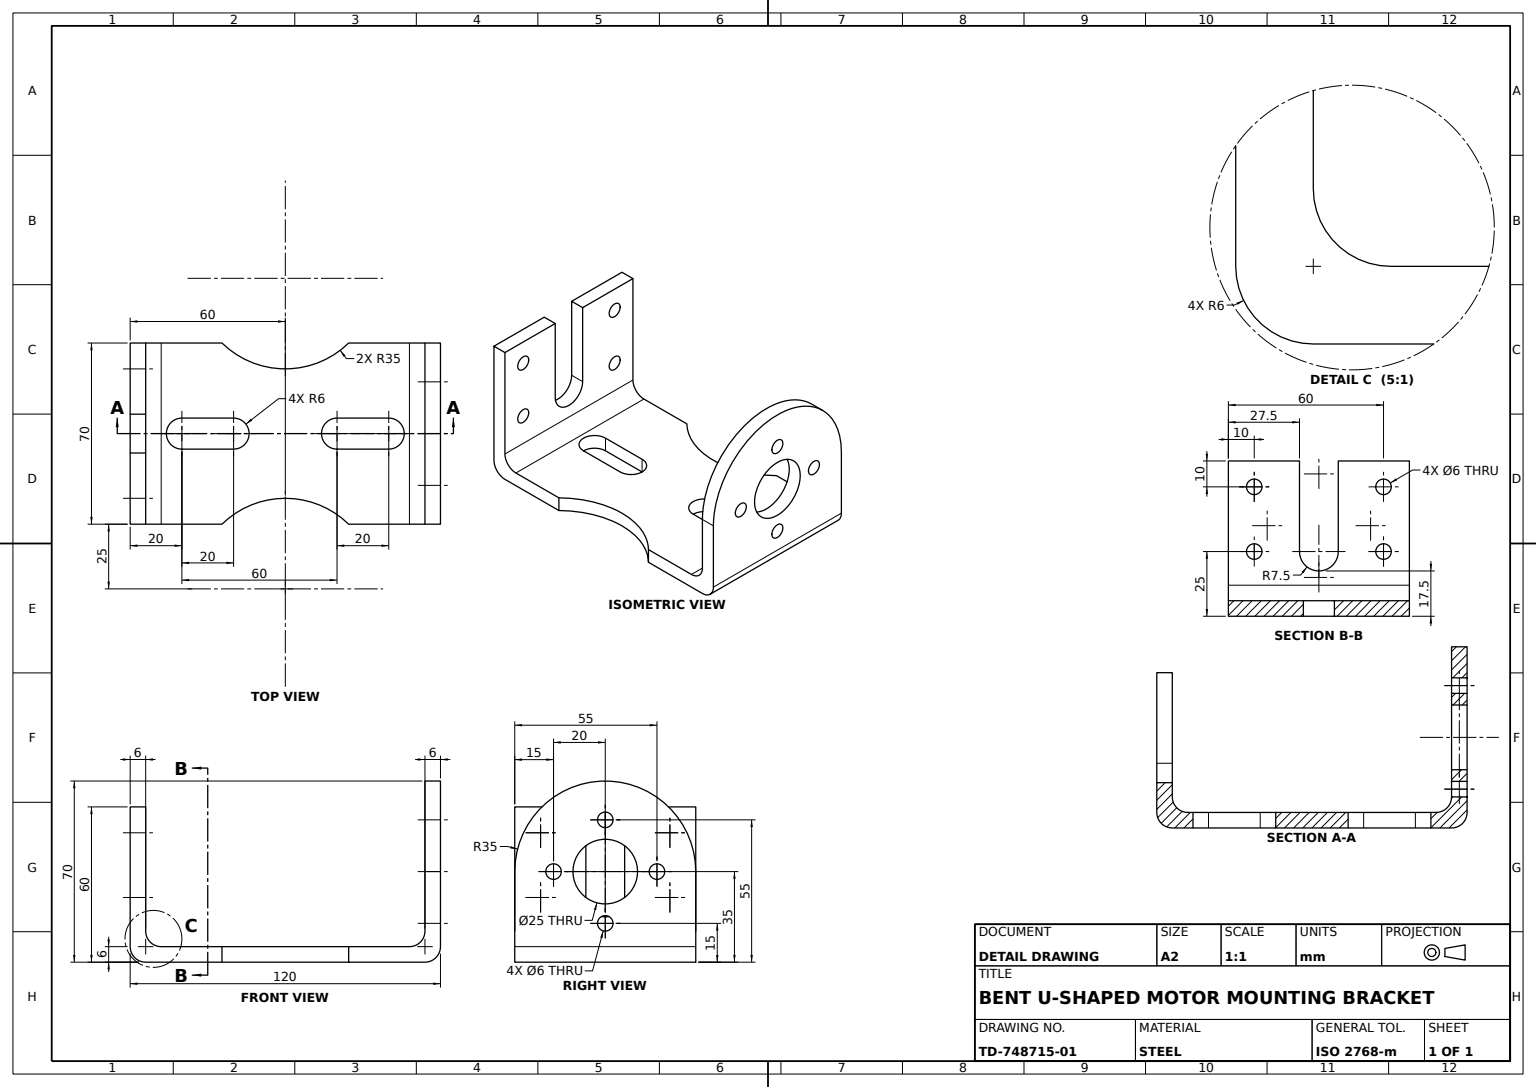
ISO-10303-21;
HEADER;
FILE_DESCRIPTION((''),'2;1');
FILE_NAME('','',(''),(''),'','','');
FILE_SCHEMA(('AUTOMOTIVE_DESIGN'));
ENDSEC;
DATA;
#1=APPLICATION_CONTEXT('');
#2=PRODUCT_CONTEXT('',#1,'mechanical');
#3=PRODUCT('','','',(#2));
#4=PRODUCT_DEFINITION_FORMATION('','',#3);
#5=PRODUCT_DEFINITION_CONTEXT('',#1,'design');
#6=PRODUCT_DEFINITION('','',#4,#5);
#7=PRODUCT_DEFINITION_SHAPE('','',#6);
#8=(LENGTH_UNIT()NAMED_UNIT(*)SI_UNIT(.MILLI.,.METRE.));
#9=(NAMED_UNIT(*)PLANE_ANGLE_UNIT()SI_UNIT($,.RADIAN.));
#10=(NAMED_UNIT(*)SI_UNIT($,.STERADIAN.)SOLID_ANGLE_UNIT());
#11=UNCERTAINTY_MEASURE_WITH_UNIT(LENGTH_MEASURE(1.E-05),#8,'distance_accuracy_value','');
#12=(GEOMETRIC_REPRESENTATION_CONTEXT(3)GLOBAL_UNCERTAINTY_ASSIGNED_CONTEXT((#11))GLOBAL_UNIT_ASSIGNED_CONTEXT((#8,#9,#10))REPRESENTATION_CONTEXT('',''));
#13=CARTESIAN_POINT('',(-20.,0.,6.));
#14=VERTEX_POINT('',#13);
#15=CARTESIAN_POINT('',(-20.,0.,-6.));
#16=VERTEX_POINT('',#15);
#17=CARTESIAN_POINT('',(-20.,0.,0.));
#18=DIRECTION('',(0.,1.,0.));
#19=DIRECTION('',(0.,0.,1.));
#20=AXIS2_PLACEMENT_3D('',#17,#18,#19);
#21=CIRCLE('',#20,6.);
#22=EDGE_CURVE('',#14,#16,#21,.T.);
#23=ORIENTED_EDGE('',*,*,#22,.T.);
#24=CARTESIAN_POINT('',(-40.,0.,-6.));
#25=VERTEX_POINT('',#24);
#26=DIRECTION('',(-1.,0.,0.));
#27=VECTOR('',#26,1000.);
#28=LINE('',#24,#27);
#29=EDGE_CURVE('',#16,#25,#28,.T.);
#30=ORIENTED_EDGE('',*,*,#29,.T.);
#31=CARTESIAN_POINT('',(-40.,0.,6.));
#32=VERTEX_POINT('',#31);
#33=CARTESIAN_POINT('',(-40.,0.,0.));
#34=AXIS2_PLACEMENT_3D('',#33,#18,#19);
#35=CIRCLE('',#34,6.);
#36=EDGE_CURVE('',#25,#32,#35,.T.);
#37=ORIENTED_EDGE('',*,*,#36,.T.);
#38=DIRECTION('',(1.,0.,0.));
#39=VECTOR('',#38,1000.);
#40=LINE('',#31,#39);
#41=EDGE_CURVE('',#32,#14,#40,.T.);
#42=ORIENTED_EDGE('',*,*,#41,.T.);
#43=EDGE_LOOP('',(#23,#30,#37,#42));
#44=FACE_BOUND('',#43,.T.);
#45=CARTESIAN_POINT('',(-54.,0.,35.));
#46=VERTEX_POINT('',#45);
#47=CARTESIAN_POINT('',(-24.494897,0.,35.));
#48=VERTEX_POINT('',#47);
#49=CARTESIAN_POINT('',(-60.,0.,35.));
#50=LINE('',#49,#39);
#51=EDGE_CURVE('',#46,#48,#50,.T.);
#52=ORIENTED_EDGE('',*,*,#51,.F.);
#53=CARTESIAN_POINT('',(-54.,0.,-35.));
#54=VERTEX_POINT('',#53);
#55=CARTESIAN_POINT('',(-54.,0.,60.));
#56=DIRECTION('',(0.,0.,-1.));
#57=VECTOR('',#56,1000.);
#58=LINE('',#55,#57);
#59=EDGE_CURVE('',#46,#54,#58,.T.);
#60=ORIENTED_EDGE('',*,*,#59,.T.);
#61=CARTESIAN_POINT('',(-24.494897,0.,-35.));
#62=VERTEX_POINT('',#61);
#63=CARTESIAN_POINT('',(-60.,0.,-35.));
#64=LINE('',#63,#27);
#65=EDGE_CURVE('',#62,#54,#64,.T.);
#66=ORIENTED_EDGE('',*,*,#65,.F.);
#67=CARTESIAN_POINT('',(24.494897,0.,-35.));
#68=VERTEX_POINT('',#67);
#69=CARTESIAN_POINT('',(0.,0.,-60.));
#70=DIRECTION('',(0.,-1.,0.));
#71=AXIS2_PLACEMENT_3D('',#69,#70,#19);
#72=CIRCLE('',#71,35.);
#73=EDGE_CURVE('',#68,#62,#72,.T.);
#74=ORIENTED_EDGE('',*,*,#73,.F.);
#75=CARTESIAN_POINT('',(54.,0.,-35.));
#76=VERTEX_POINT('',#75);
#77=LINE('',#67,#27);
#78=EDGE_CURVE('',#76,#68,#77,.T.);
#79=ORIENTED_EDGE('',*,*,#78,.F.);
#80=CARTESIAN_POINT('',(54.,0.,35.));
#81=VERTEX_POINT('',#80);
#82=CARTESIAN_POINT('',(54.,0.,60.));
#83=VECTOR('',#19,1000.);
#84=LINE('',#82,#83);
#85=EDGE_CURVE('',#76,#81,#84,.T.);
#86=ORIENTED_EDGE('',*,*,#85,.T.);
#87=CARTESIAN_POINT('',(24.494897,0.,35.));
#88=VERTEX_POINT('',#87);
#89=LINE('',#87,#39);
#90=EDGE_CURVE('',#88,#81,#89,.T.);
#91=ORIENTED_EDGE('',*,*,#90,.F.);
#92=CARTESIAN_POINT('',(0.,0.,25.));
#93=VERTEX_POINT('',#92);
#94=CARTESIAN_POINT('',(0.,0.,60.));
#95=AXIS2_PLACEMENT_3D('',#94,#70,#19);
#96=CIRCLE('',#95,35.);
#97=EDGE_CURVE('',#93,#88,#96,.T.);
#98=ORIENTED_EDGE('',*,*,#97,.F.);
#99=EDGE_CURVE('',#48,#93,#96,.T.);
#100=ORIENTED_EDGE('',*,*,#99,.F.);
#101=EDGE_LOOP('',(#52,#60,#66,#74,#79,#86,#91,#98,#100));
#102=FACE_OUTER_BOUND('',#101,.T.);
#103=CARTESIAN_POINT('',(20.,0.,6.));
#104=VERTEX_POINT('',#103);
#105=CARTESIAN_POINT('',(40.,0.,6.));
#106=VERTEX_POINT('',#105);
#107=LINE('',#103,#39);
#108=EDGE_CURVE('',#104,#106,#107,.T.);
#109=ORIENTED_EDGE('',*,*,#108,.T.);
#110=CARTESIAN_POINT('',(40.,0.,-6.));
#111=VERTEX_POINT('',#110);
#112=CARTESIAN_POINT('',(40.,0.,0.));
#113=AXIS2_PLACEMENT_3D('',#112,#18,#19);
#114=CIRCLE('',#113,6.);
#115=EDGE_CURVE('',#106,#111,#114,.T.);
#116=ORIENTED_EDGE('',*,*,#115,.T.);
#117=CARTESIAN_POINT('',(20.,0.,-6.));
#118=VERTEX_POINT('',#117);
#119=LINE('',#117,#27);
#120=EDGE_CURVE('',#111,#118,#119,.T.);
#121=ORIENTED_EDGE('',*,*,#120,.T.);
#122=CARTESIAN_POINT('',(20.,0.,0.));
#123=AXIS2_PLACEMENT_3D('',#122,#18,#19);
#124=CIRCLE('',#123,6.);
#125=EDGE_CURVE('',#118,#104,#124,.T.);
#126=ORIENTED_EDGE('',*,*,#125,.T.);
#127=EDGE_LOOP('',(#109,#116,#121,#126));
#128=FACE_BOUND('',#127,.T.);
#129=AXIS2_PLACEMENT_3D('',#94,#18,#19);
#130=PLANE('',#129);
#131=ADVANCED_FACE('',(#44,#102,#128),#130,.F.);
#132=CARTESIAN_POINT('',(60.,35.,-12.5));
#133=VERTEX_POINT('',#132);
#134=CARTESIAN_POINT('',(60.,35.,12.5));
#135=VERTEX_POINT('',#134);
#136=CARTESIAN_POINT('',(60.,35.,0.));
#137=AXIS2_PLACEMENT_3D('',#136,#38,#56);
#138=CIRCLE('',#137,12.5);
#139=EDGE_CURVE('',#133,#135,#138,.T.);
#140=ORIENTED_EDGE('',*,*,#139,.T.);
#141=CARTESIAN_POINT('',(54.,35.,12.5));
#142=VERTEX_POINT('',#141);
#143=LINE('',#141,#39);
#144=EDGE_CURVE('',#142,#135,#143,.T.);
#145=ORIENTED_EDGE('',*,*,#144,.F.);
#146=CARTESIAN_POINT('',(54.,35.,-12.5));
#147=VERTEX_POINT('',#146);
#148=CARTESIAN_POINT('',(54.,35.,0.));
#149=AXIS2_PLACEMENT_3D('',#148,#38,#56);
#150=CIRCLE('',#149,12.5);
#151=EDGE_CURVE('',#147,#142,#150,.T.);
#152=ORIENTED_EDGE('',*,*,#151,.F.);
#153=LINE('',#146,#39);
#154=EDGE_CURVE('',#147,#133,#153,.T.);
#155=ORIENTED_EDGE('',*,*,#154,.T.);
#156=EDGE_LOOP('',(#140,#145,#152,#155));
#157=FACE_OUTER_BOUND('',#156,.T.);
#158=CYLINDRICAL_SURFACE('',#149,12.5);
#159=ADVANCED_FACE('',(#157),#158,.F.);
#160=CARTESIAN_POINT('',(-40.,6.,-6.));
#161=VERTEX_POINT('',#160);
#162=CARTESIAN_POINT('',(-40.,6.,6.));
#163=VERTEX_POINT('',#162);
#164=CARTESIAN_POINT('',(-40.,6.,0.));
#165=AXIS2_PLACEMENT_3D('',#164,#18,#19);
#166=CIRCLE('',#165,6.);
#167=EDGE_CURVE('',#161,#163,#166,.T.);
#168=ORIENTED_EDGE('',*,*,#167,.T.);
#169=VECTOR('',#70,1000.);
#170=LINE('',#162,#169);
#171=EDGE_CURVE('',#163,#32,#170,.T.);
#172=ORIENTED_EDGE('',*,*,#171,.T.);
#173=ORIENTED_EDGE('',*,*,#36,.F.);
#174=LINE('',#160,#169);
#175=EDGE_CURVE('',#161,#25,#174,.T.);
#176=ORIENTED_EDGE('',*,*,#175,.F.);
#177=EDGE_LOOP('',(#168,#172,#173,#176));
#178=FACE_OUTER_BOUND('',#177,.T.);
#179=AXIS2_PLACEMENT_3D('',#164,#70,#56);
#180=CYLINDRICAL_SURFACE('',#179,6.);
#181=ADVANCED_FACE('',(#178),#180,.F.);
#182=CARTESIAN_POINT('',(54.,35.,-23.));
#183=VERTEX_POINT('',#182);
#184=CARTESIAN_POINT('',(54.,35.,-17.));
#185=VERTEX_POINT('',#184);
#186=CARTESIAN_POINT('',(54.,35.,-20.));
#187=AXIS2_PLACEMENT_3D('',#186,#38,#56);
#188=CIRCLE('',#187,3.);
#189=EDGE_CURVE('',#183,#185,#188,.T.);
#190=ORIENTED_EDGE('',*,*,#189,.F.);
#191=CARTESIAN_POINT('',(60.,35.,-23.));
#192=VERTEX_POINT('',#191);
#193=LINE('',#182,#39);
#194=EDGE_CURVE('',#183,#192,#193,.T.);
#195=ORIENTED_EDGE('',*,*,#194,.T.);
#196=CARTESIAN_POINT('',(60.,35.,-17.));
#197=VERTEX_POINT('',#196);
#198=CARTESIAN_POINT('',(60.,35.,-20.));
#199=AXIS2_PLACEMENT_3D('',#198,#38,#56);
#200=CIRCLE('',#199,3.);
#201=EDGE_CURVE('',#192,#197,#200,.T.);
#202=ORIENTED_EDGE('',*,*,#201,.T.);
#203=LINE('',#184,#39);
#204=EDGE_CURVE('',#185,#197,#203,.T.);
#205=ORIENTED_EDGE('',*,*,#204,.F.);
#206=EDGE_LOOP('',(#190,#195,#202,#205));
#207=FACE_OUTER_BOUND('',#206,.T.);
#208=CYLINDRICAL_SURFACE('',#187,3.);
#209=ADVANCED_FACE('',(#207),#208,.F.);
#210=CARTESIAN_POINT('',(-60.,50.,22.));
#211=VERTEX_POINT('',#210);
#212=CARTESIAN_POINT('',(-60.,50.,28.));
#213=VERTEX_POINT('',#212);
#214=CARTESIAN_POINT('',(-60.,50.,25.));
#215=AXIS2_PLACEMENT_3D('',#214,#26,#19);
#216=CIRCLE('',#215,3.);
#217=EDGE_CURVE('',#211,#213,#216,.T.);
#218=ORIENTED_EDGE('',*,*,#217,.T.);
#219=CARTESIAN_POINT('',(-54.,50.,28.));
#220=VERTEX_POINT('',#219);
#221=LINE('',#219,#27);
#222=EDGE_CURVE('',#220,#213,#221,.T.);
#223=ORIENTED_EDGE('',*,*,#222,.F.);
#224=CARTESIAN_POINT('',(-54.,50.,22.));
#225=VERTEX_POINT('',#224);
#226=CARTESIAN_POINT('',(-54.,50.,25.));
#227=AXIS2_PLACEMENT_3D('',#226,#26,#19);
#228=CIRCLE('',#227,3.);
#229=EDGE_CURVE('',#225,#220,#228,.T.);
#230=ORIENTED_EDGE('',*,*,#229,.F.);
#231=LINE('',#224,#27);
#232=EDGE_CURVE('',#225,#211,#231,.T.);
#233=ORIENTED_EDGE('',*,*,#232,.T.);
#234=EDGE_LOOP('',(#218,#223,#230,#233));
#235=FACE_OUTER_BOUND('',#234,.T.);
#236=CYLINDRICAL_SURFACE('',#227,3.);
#237=ADVANCED_FACE('',(#235),#236,.F.);
#238=CARTESIAN_POINT('',(20.,6.,6.));
#239=VERTEX_POINT('',#238);
#240=LINE('',#238,#169);
#241=EDGE_CURVE('',#239,#104,#240,.T.);
#242=ORIENTED_EDGE('',*,*,#241,.T.);
#243=ORIENTED_EDGE('',*,*,#125,.F.);
#244=CARTESIAN_POINT('',(20.,6.,-6.));
#245=VERTEX_POINT('',#244);
#246=LINE('',#244,#169);
#247=EDGE_CURVE('',#245,#118,#246,.T.);
#248=ORIENTED_EDGE('',*,*,#247,.F.);
#249=CARTESIAN_POINT('',(20.,6.,0.));
#250=AXIS2_PLACEMENT_3D('',#249,#18,#19);
#251=CIRCLE('',#250,6.);
#252=EDGE_CURVE('',#245,#239,#251,.T.);
#253=ORIENTED_EDGE('',*,*,#252,.T.);
#254=EDGE_LOOP('',(#242,#243,#248,#253));
#255=FACE_OUTER_BOUND('',#254,.T.);
#256=AXIS2_PLACEMENT_3D('',#249,#70,#56);
#257=CYLINDRICAL_SURFACE('',#256,6.);
#258=ADVANCED_FACE('',(#255),#257,.F.);
#259=CARTESIAN_POINT('',(60.,55.,3.));
#260=VERTEX_POINT('',#259);
#261=CARTESIAN_POINT('',(60.,55.,-3.));
#262=VERTEX_POINT('',#261);
#263=CARTESIAN_POINT('',(60.,55.,0.));
#264=AXIS2_PLACEMENT_3D('',#263,#38,#56);
#265=CIRCLE('',#264,3.);
#266=EDGE_CURVE('',#260,#262,#265,.T.);
#267=ORIENTED_EDGE('',*,*,#266,.T.);
#268=CARTESIAN_POINT('',(54.,55.,-3.));
#269=VERTEX_POINT('',#268);
#270=LINE('',#268,#39);
#271=EDGE_CURVE('',#269,#262,#270,.T.);
#272=ORIENTED_EDGE('',*,*,#271,.F.);
#273=CARTESIAN_POINT('',(54.,55.,3.));
#274=VERTEX_POINT('',#273);
#275=CARTESIAN_POINT('',(54.,55.,0.));
#276=AXIS2_PLACEMENT_3D('',#275,#38,#56);
#277=CIRCLE('',#276,3.);
#278=EDGE_CURVE('',#274,#269,#277,.T.);
#279=ORIENTED_EDGE('',*,*,#278,.F.);
#280=LINE('',#273,#39);
#281=EDGE_CURVE('',#274,#260,#280,.T.);
#282=ORIENTED_EDGE('',*,*,#281,.T.);
#283=EDGE_LOOP('',(#267,#272,#279,#282));
#284=FACE_OUTER_BOUND('',#283,.T.);
#285=CYLINDRICAL_SURFACE('',#276,3.);
#286=ADVANCED_FACE('',(#284),#285,.F.);
#287=CARTESIAN_POINT('',(-54.,25.,22.));
#288=VERTEX_POINT('',#287);
#289=CARTESIAN_POINT('',(-60.,25.,22.));
#290=VERTEX_POINT('',#289);
#291=LINE('',#287,#27);
#292=EDGE_CURVE('',#288,#290,#291,.T.);
#293=ORIENTED_EDGE('',*,*,#292,.T.);
#294=CARTESIAN_POINT('',(-60.,25.,28.));
#295=VERTEX_POINT('',#294);
#296=CARTESIAN_POINT('',(-60.,25.,25.));
#297=AXIS2_PLACEMENT_3D('',#296,#26,#19);
#298=CIRCLE('',#297,3.);
#299=EDGE_CURVE('',#290,#295,#298,.T.);
#300=ORIENTED_EDGE('',*,*,#299,.T.);
#301=CARTESIAN_POINT('',(-54.,25.,28.));
#302=VERTEX_POINT('',#301);
#303=LINE('',#301,#27);
#304=EDGE_CURVE('',#302,#295,#303,.T.);
#305=ORIENTED_EDGE('',*,*,#304,.F.);
#306=CARTESIAN_POINT('',(-54.,25.,25.));
#307=AXIS2_PLACEMENT_3D('',#306,#26,#19);
#308=CIRCLE('',#307,3.);
#309=EDGE_CURVE('',#288,#302,#308,.T.);
#310=ORIENTED_EDGE('',*,*,#309,.F.);
#311=EDGE_LOOP('',(#293,#300,#305,#310));
#312=FACE_OUTER_BOUND('',#311,.T.);
#313=CYLINDRICAL_SURFACE('',#307,3.);
#314=ADVANCED_FACE('',(#312),#313,.F.);
#315=EDGE_CURVE('',#220,#225,#228,.T.);
#316=ORIENTED_EDGE('',*,*,#315,.F.);
#317=ORIENTED_EDGE('',*,*,#222,.T.);
#318=EDGE_CURVE('',#213,#211,#216,.T.);
#319=ORIENTED_EDGE('',*,*,#318,.T.);
#320=ORIENTED_EDGE('',*,*,#232,.F.);
#321=EDGE_LOOP('',(#316,#317,#319,#320));
#322=FACE_OUTER_BOUND('',#321,.T.);
#323=ADVANCED_FACE('',(#322),#236,.F.);
#324=ORIENTED_EDGE('',*,*,#292,.F.);
#325=EDGE_CURVE('',#302,#288,#308,.T.);
#326=ORIENTED_EDGE('',*,*,#325,.F.);
#327=ORIENTED_EDGE('',*,*,#304,.T.);
#328=EDGE_CURVE('',#295,#290,#298,.T.);
#329=ORIENTED_EDGE('',*,*,#328,.T.);
#330=EDGE_LOOP('',(#324,#326,#327,#329));
#331=FACE_OUTER_BOUND('',#330,.T.);
#332=ADVANCED_FACE('',(#331),#313,.F.);
#333=CARTESIAN_POINT('',(-60.,25.,-7.5));
#334=VERTEX_POINT('',#333);
#335=CARTESIAN_POINT('',(-60.,60.,-7.5));
#336=VERTEX_POINT('',#335);
#337=CARTESIAN_POINT('',(-60.,0.,-7.5));
#338=VECTOR('',#18,1000.);
#339=LINE('',#337,#338);
#340=EDGE_CURVE('',#334,#336,#339,.T.);
#341=ORIENTED_EDGE('',*,*,#340,.F.);
#342=CARTESIAN_POINT('',(-54.,25.,-7.5));
#343=VERTEX_POINT('',#342);
#344=LINE('',#342,#27);
#345=EDGE_CURVE('',#343,#334,#344,.T.);
#346=ORIENTED_EDGE('',*,*,#345,.F.);
#347=CARTESIAN_POINT('',(-54.,60.,-7.5));
#348=VERTEX_POINT('',#347);
#349=CARTESIAN_POINT('',(-54.,0.,-7.5));
#350=LINE('',#349,#338);
#351=EDGE_CURVE('',#343,#348,#350,.T.);
#352=ORIENTED_EDGE('',*,*,#351,.T.);
#353=LINE('',#347,#27);
#354=EDGE_CURVE('',#348,#336,#353,.T.);
#355=ORIENTED_EDGE('',*,*,#354,.T.);
#356=EDGE_LOOP('',(#341,#346,#352,#355));
#357=FACE_OUTER_BOUND('',#356,.T.);
#358=AXIS2_PLACEMENT_3D('',#349,#19,#70);
#359=PLANE('',#358);
#360=ADVANCED_FACE('',(#357),#359,.T.);
#361=CARTESIAN_POINT('',(-60.,50.,-22.));
#362=VERTEX_POINT('',#361);
#363=CARTESIAN_POINT('',(-60.,50.,-28.));
#364=VERTEX_POINT('',#363);
#365=CARTESIAN_POINT('',(-60.,50.,-25.));
#366=AXIS2_PLACEMENT_3D('',#365,#26,#19);
#367=CIRCLE('',#366,3.);
#368=EDGE_CURVE('',#362,#364,#367,.T.);
#369=ORIENTED_EDGE('',*,*,#368,.F.);
#370=EDGE_CURVE('',#364,#362,#367,.T.);
#371=ORIENTED_EDGE('',*,*,#370,.F.);
#372=EDGE_LOOP('',(#369,#371));
#373=FACE_BOUND('',#372,.T.);
#374=CARTESIAN_POINT('',(-60.,25.,-22.));
#375=VERTEX_POINT('',#374);
#376=CARTESIAN_POINT('',(-60.,25.,-28.));
#377=VERTEX_POINT('',#376);
#378=CARTESIAN_POINT('',(-60.,25.,-25.));
#379=AXIS2_PLACEMENT_3D('',#378,#26,#19);
#380=CIRCLE('',#379,3.);
#381=EDGE_CURVE('',#375,#377,#380,.T.);
#382=ORIENTED_EDGE('',*,*,#381,.F.);
#383=EDGE_CURVE('',#377,#375,#380,.T.);
#384=ORIENTED_EDGE('',*,*,#383,.F.);
#385=EDGE_LOOP('',(#382,#384));
#386=FACE_BOUND('',#385,.T.);
#387=CARTESIAN_POINT('',(-60.,60.,-35.));
#388=VERTEX_POINT('',#387);
#389=CARTESIAN_POINT('',(-60.,60.,0.));
#390=LINE('',#389,#83);
#391=EDGE_CURVE('',#388,#336,#390,.T.);
#392=ORIENTED_EDGE('',*,*,#391,.F.);
#393=CARTESIAN_POINT('',(-60.,6.,-35.));
#394=VERTEX_POINT('',#393);
#395=LINE('',#393,#169);
#396=EDGE_CURVE('',#388,#394,#395,.T.);
#397=ORIENTED_EDGE('',*,*,#396,.T.);
#398=CARTESIAN_POINT('',(-60.,6.,35.));
#399=VERTEX_POINT('',#398);
#400=LINE('',#393,#83);
#401=EDGE_CURVE('',#394,#399,#400,.T.);
#402=ORIENTED_EDGE('',*,*,#401,.T.);
#403=CARTESIAN_POINT('',(-60.,60.,35.));
#404=VERTEX_POINT('',#403);
#405=LINE('',#398,#169);
#406=EDGE_CURVE('',#404,#399,#405,.T.);
#407=ORIENTED_EDGE('',*,*,#406,.F.);
#408=CARTESIAN_POINT('',(-60.,60.,7.5));
#409=VERTEX_POINT('',#408);
#410=LINE('',#389,#57);
#411=EDGE_CURVE('',#404,#409,#410,.T.);
#412=ORIENTED_EDGE('',*,*,#411,.T.);
#413=CARTESIAN_POINT('',(-60.,25.,7.5));
#414=VERTEX_POINT('',#413);
#415=CARTESIAN_POINT('',(-60.,0.,7.5));
#416=LINE('',#415,#338);
#417=EDGE_CURVE('',#414,#409,#416,.T.);
#418=ORIENTED_EDGE('',*,*,#417,.F.);
#419=CARTESIAN_POINT('',(-60.,25.,0.));
#420=AXIS2_PLACEMENT_3D('',#419,#26,#19);
#421=CIRCLE('',#420,7.5);
#422=EDGE_CURVE('',#334,#414,#421,.T.);
#423=ORIENTED_EDGE('',*,*,#422,.F.);
#424=ORIENTED_EDGE('',*,*,#340,.T.);
#425=EDGE_LOOP('',(#392,#397,#402,#407,#412,#418,#423,#424));
#426=FACE_OUTER_BOUND('',#425,.T.);
#427=ORIENTED_EDGE('',*,*,#299,.F.);
#428=ORIENTED_EDGE('',*,*,#328,.F.);
#429=EDGE_LOOP('',(#427,#428));
#430=FACE_BOUND('',#429,.T.);
#431=ORIENTED_EDGE('',*,*,#318,.F.);
#432=ORIENTED_EDGE('',*,*,#217,.F.);
#433=EDGE_LOOP('',(#431,#432));
#434=FACE_BOUND('',#433,.T.);
#435=AXIS2_PLACEMENT_3D('',#393,#38,#56);
#436=PLANE('',#435);
#437=ADVANCED_FACE('',(#373,#386,#426,#430,#434),#436,.F.);
#438=CARTESIAN_POINT('',(-54.,12.,35.));
#439=VERTEX_POINT('',#438);
#440=CARTESIAN_POINT('',(-54.,12.,-35.));
#441=VERTEX_POINT('',#440);
#442=CARTESIAN_POINT('',(-54.,12.,0.));
#443=LINE('',#442,#57);
#444=EDGE_CURVE('',#439,#441,#443,.T.);
#445=ORIENTED_EDGE('',*,*,#444,.T.);
#446=CARTESIAN_POINT('',(-54.,60.,-35.));
#447=VERTEX_POINT('',#446);
#448=LINE('',#53,#338);
#449=EDGE_CURVE('',#441,#447,#448,.T.);
#450=ORIENTED_EDGE('',*,*,#449,.T.);
#451=CARTESIAN_POINT('',(-54.,60.,0.));
#452=LINE('',#451,#83);
#453=EDGE_CURVE('',#447,#348,#452,.T.);
#454=ORIENTED_EDGE('',*,*,#453,.T.);
#455=ORIENTED_EDGE('',*,*,#351,.F.);
#456=CARTESIAN_POINT('',(-54.,25.,7.5));
#457=VERTEX_POINT('',#456);
#458=CARTESIAN_POINT('',(-54.,25.,0.));
#459=AXIS2_PLACEMENT_3D('',#458,#26,#19);
#460=CIRCLE('',#459,7.5);
#461=EDGE_CURVE('',#343,#457,#460,.T.);
#462=ORIENTED_EDGE('',*,*,#461,.T.);
#463=CARTESIAN_POINT('',(-54.,60.,7.5));
#464=VERTEX_POINT('',#463);
#465=CARTESIAN_POINT('',(-54.,0.,7.5));
#466=LINE('',#465,#338);
#467=EDGE_CURVE('',#457,#464,#466,.T.);
#468=ORIENTED_EDGE('',*,*,#467,.T.);
#469=CARTESIAN_POINT('',(-54.,60.,35.));
#470=VERTEX_POINT('',#469);
#471=LINE('',#451,#57);
#472=EDGE_CURVE('',#470,#464,#471,.T.);
#473=ORIENTED_EDGE('',*,*,#472,.F.);
#474=LINE('',#45,#338);
#475=EDGE_CURVE('',#439,#470,#474,.T.);
#476=ORIENTED_EDGE('',*,*,#475,.F.);
#477=EDGE_LOOP('',(#445,#450,#454,#455,#462,#468,#473,#476));
#478=FACE_OUTER_BOUND('',#477,.T.);
#479=ORIENTED_EDGE('',*,*,#229,.T.);
#480=ORIENTED_EDGE('',*,*,#315,.T.);
#481=EDGE_LOOP('',(#479,#480));
#482=FACE_BOUND('',#481,.T.);
#483=CARTESIAN_POINT('',(-54.,25.,-28.));
#484=VERTEX_POINT('',#483);
#485=CARTESIAN_POINT('',(-54.,25.,-22.));
#486=VERTEX_POINT('',#485);
#487=CARTESIAN_POINT('',(-54.,25.,-25.));
#488=AXIS2_PLACEMENT_3D('',#487,#26,#19);
#489=CIRCLE('',#488,3.);
#490=EDGE_CURVE('',#484,#486,#489,.T.);
#491=ORIENTED_EDGE('',*,*,#490,.T.);
#492=EDGE_CURVE('',#486,#484,#489,.T.);
#493=ORIENTED_EDGE('',*,*,#492,.T.);
#494=EDGE_LOOP('',(#491,#493));
#495=FACE_BOUND('',#494,.T.);
#496=CARTESIAN_POINT('',(-54.,50.,-22.));
#497=VERTEX_POINT('',#496);
#498=CARTESIAN_POINT('',(-54.,50.,-28.));
#499=VERTEX_POINT('',#498);
#500=CARTESIAN_POINT('',(-54.,50.,-25.));
#501=AXIS2_PLACEMENT_3D('',#500,#26,#19);
#502=CIRCLE('',#501,3.);
#503=EDGE_CURVE('',#497,#499,#502,.T.);
#504=ORIENTED_EDGE('',*,*,#503,.T.);
#505=EDGE_CURVE('',#499,#497,#502,.T.);
#506=ORIENTED_EDGE('',*,*,#505,.T.);
#507=EDGE_LOOP('',(#504,#506));
#508=FACE_BOUND('',#507,.T.);
#509=ORIENTED_EDGE('',*,*,#325,.T.);
#510=ORIENTED_EDGE('',*,*,#309,.T.);
#511=EDGE_LOOP('',(#509,#510));
#512=FACE_BOUND('',#511,.T.);
#513=CARTESIAN_POINT('',(-54.,0.,0.));
#514=AXIS2_PLACEMENT_3D('',#513,#26,#19);
#515=PLANE('',#514);
#516=ADVANCED_FACE('',(#478,#482,#495,#508,#512),#515,.F.);
#517=CARTESIAN_POINT('',(40.,6.,-6.));
#518=VERTEX_POINT('',#517);
#519=LINE('',#244,#27);
#520=EDGE_CURVE('',#518,#245,#519,.T.);
#521=ORIENTED_EDGE('',*,*,#520,.T.);
#522=ORIENTED_EDGE('',*,*,#247,.T.);
#523=ORIENTED_EDGE('',*,*,#120,.F.);
#524=LINE('',#517,#169);
#525=EDGE_CURVE('',#518,#111,#524,.T.);
#526=ORIENTED_EDGE('',*,*,#525,.F.);
#527=EDGE_LOOP('',(#521,#522,#523,#526));
#528=FACE_OUTER_BOUND('',#527,.T.);
#529=AXIS2_PLACEMENT_3D('',#244,#19,#38);
#530=PLANE('',#529);
#531=ADVANCED_FACE('',(#528),#530,.T.);
#532=CARTESIAN_POINT('',(60.,6.,35.));
#533=VERTEX_POINT('',#532);
#534=CARTESIAN_POINT('',(60.,6.,-35.));
#535=VERTEX_POINT('',#534);
#536=LINE('',#534,#57);
#537=EDGE_CURVE('',#533,#535,#536,.T.);
#538=ORIENTED_EDGE('',*,*,#537,.T.);
#539=CARTESIAN_POINT('',(60.,35.,-35.));
#540=VERTEX_POINT('',#539);
#541=LINE('',#534,#169);
#542=EDGE_CURVE('',#540,#535,#541,.T.);
#543=ORIENTED_EDGE('',*,*,#542,.F.);
#544=CARTESIAN_POINT('',(60.,35.,35.));
#545=VERTEX_POINT('',#544);
#546=AXIS2_PLACEMENT_3D('',#136,#38,#19);
#547=CIRCLE('',#546,35.);
#548=EDGE_CURVE('',#540,#545,#547,.T.);
#549=ORIENTED_EDGE('',*,*,#548,.T.);
#550=LINE('',#532,#169);
#551=EDGE_CURVE('',#545,#533,#550,.T.);
#552=ORIENTED_EDGE('',*,*,#551,.T.);
#553=EDGE_LOOP('',(#538,#543,#549,#552));
#554=FACE_OUTER_BOUND('',#553,.T.);
#555=ORIENTED_EDGE('',*,*,#266,.F.);
#556=EDGE_CURVE('',#262,#260,#265,.T.);
#557=ORIENTED_EDGE('',*,*,#556,.F.);
#558=EDGE_LOOP('',(#555,#557));
#559=FACE_BOUND('',#558,.T.);
#560=EDGE_CURVE('',#197,#192,#200,.T.);
#561=ORIENTED_EDGE('',*,*,#560,.F.);
#562=ORIENTED_EDGE('',*,*,#201,.F.);
#563=EDGE_LOOP('',(#561,#562));
#564=FACE_BOUND('',#563,.T.);
#565=EDGE_CURVE('',#135,#133,#138,.T.);
#566=ORIENTED_EDGE('',*,*,#565,.F.);
#567=ORIENTED_EDGE('',*,*,#139,.F.);
#568=EDGE_LOOP('',(#566,#567));
#569=FACE_BOUND('',#568,.T.);
#570=CARTESIAN_POINT('',(60.,15.,-3.));
#571=VERTEX_POINT('',#570);
#572=CARTESIAN_POINT('',(60.,15.,3.));
#573=VERTEX_POINT('',#572);
#574=CARTESIAN_POINT('',(60.,15.,0.));
#575=AXIS2_PLACEMENT_3D('',#574,#38,#56);
#576=CIRCLE('',#575,3.);
#577=EDGE_CURVE('',#571,#573,#576,.T.);
#578=ORIENTED_EDGE('',*,*,#577,.F.);
#579=EDGE_CURVE('',#573,#571,#576,.T.);
#580=ORIENTED_EDGE('',*,*,#579,.F.);
#581=EDGE_LOOP('',(#578,#580));
#582=FACE_BOUND('',#581,.T.);
#583=CARTESIAN_POINT('',(60.,35.,17.));
#584=VERTEX_POINT('',#583);
#585=CARTESIAN_POINT('',(60.,35.,23.));
#586=VERTEX_POINT('',#585);
#587=CARTESIAN_POINT('',(60.,35.,20.));
#588=AXIS2_PLACEMENT_3D('',#587,#38,#56);
#589=CIRCLE('',#588,3.);
#590=EDGE_CURVE('',#584,#586,#589,.T.);
#591=ORIENTED_EDGE('',*,*,#590,.F.);
#592=EDGE_CURVE('',#586,#584,#589,.T.);
#593=ORIENTED_EDGE('',*,*,#592,.F.);
#594=EDGE_LOOP('',(#591,#593));
#595=FACE_BOUND('',#594,.T.);
#596=AXIS2_PLACEMENT_3D('',#534,#26,#19);
#597=PLANE('',#596);
#598=ADVANCED_FACE('',(#554,#559,#564,#569,#582,#595),#597,.F.);
#599=CARTESIAN_POINT('',(40.,6.,6.));
#600=VERTEX_POINT('',#599);
#601=LINE('',#599,#169);
#602=EDGE_CURVE('',#600,#106,#601,.T.);
#603=ORIENTED_EDGE('',*,*,#602,.T.);
#604=ORIENTED_EDGE('',*,*,#108,.F.);
#605=ORIENTED_EDGE('',*,*,#241,.F.);
#606=LINE('',#238,#39);
#607=EDGE_CURVE('',#239,#600,#606,.T.);
#608=ORIENTED_EDGE('',*,*,#607,.T.);
#609=EDGE_LOOP('',(#603,#604,#605,#608));
#610=FACE_OUTER_BOUND('',#609,.T.);
#611=AXIS2_PLACEMENT_3D('',#238,#56,#26);
#612=PLANE('',#611);
#613=ADVANCED_FACE('',(#610),#612,.T.);
#614=ORIENTED_EDGE('',*,*,#417,.T.);
#615=LINE('',#463,#27);
#616=EDGE_CURVE('',#464,#409,#615,.T.);
#617=ORIENTED_EDGE('',*,*,#616,.F.);
#618=ORIENTED_EDGE('',*,*,#467,.F.);
#619=LINE('',#456,#27);
#620=EDGE_CURVE('',#457,#414,#619,.T.);
#621=ORIENTED_EDGE('',*,*,#620,.T.);
#622=EDGE_LOOP('',(#614,#617,#618,#621));
#623=FACE_OUTER_BOUND('',#622,.T.);
#624=AXIS2_PLACEMENT_3D('',#465,#19,#70);
#625=PLANE('',#624);
#626=ADVANCED_FACE('',(#623),#625,.F.);
#627=CARTESIAN_POINT('',(54.,15.,3.));
#628=VERTEX_POINT('',#627);
#629=LINE('',#627,#39);
#630=EDGE_CURVE('',#628,#573,#629,.T.);
#631=ORIENTED_EDGE('',*,*,#630,.T.);
#632=ORIENTED_EDGE('',*,*,#579,.T.);
#633=CARTESIAN_POINT('',(54.,15.,-3.));
#634=VERTEX_POINT('',#633);
#635=LINE('',#633,#39);
#636=EDGE_CURVE('',#634,#571,#635,.T.);
#637=ORIENTED_EDGE('',*,*,#636,.F.);
#638=CARTESIAN_POINT('',(54.,12.,0.));
#639=VERTEX_POINT('',#638);
#640=CARTESIAN_POINT('',(54.,15.,0.));
#641=AXIS2_PLACEMENT_3D('',#640,#38,#56);
#642=CIRCLE('',#641,3.);
#643=EDGE_CURVE('',#639,#634,#642,.T.);
#644=ORIENTED_EDGE('',*,*,#643,.F.);
#645=EDGE_CURVE('',#628,#639,#642,.T.);
#646=ORIENTED_EDGE('',*,*,#645,.F.);
#647=EDGE_LOOP('',(#631,#632,#637,#644,#646));
#648=FACE_OUTER_BOUND('',#647,.T.);
#649=CYLINDRICAL_SURFACE('',#641,3.);
#650=ADVANCED_FACE('',(#648),#649,.F.);
#651=ORIENTED_EDGE('',*,*,#354,.F.);
#652=ORIENTED_EDGE('',*,*,#453,.F.);
#653=LINE('',#446,#27);
#654=EDGE_CURVE('',#447,#388,#653,.T.);
#655=ORIENTED_EDGE('',*,*,#654,.T.);
#656=ORIENTED_EDGE('',*,*,#391,.T.);
#657=EDGE_LOOP('',(#651,#652,#655,#656));
#658=FACE_OUTER_BOUND('',#657,.T.);
#659=AXIS2_PLACEMENT_3D('',#451,#70,#56);
#660=PLANE('',#659);
#661=ADVANCED_FACE('',(#658),#660,.F.);
#662=CARTESIAN_POINT('',(-24.494897,6.,-35.));
#663=VERTEX_POINT('',#662);
#664=LINE('',#662,#169);
#665=EDGE_CURVE('',#663,#62,#664,.T.);
#666=ORIENTED_EDGE('',*,*,#665,.T.);
#667=ORIENTED_EDGE('',*,*,#65,.T.);
#668=CARTESIAN_POINT('',(-54.,6.,-35.));
#669=AXIS2_PLACEMENT_3D('',#668,#56,#38);
#670=CIRCLE('',#669,6.);
#671=EDGE_CURVE('',#54,#394,#670,.T.);
#672=ORIENTED_EDGE('',*,*,#671,.T.);
#673=ORIENTED_EDGE('',*,*,#396,.F.);
#674=ORIENTED_EDGE('',*,*,#654,.F.);
#675=ORIENTED_EDGE('',*,*,#449,.F.);
#676=CARTESIAN_POINT('',(-48.,6.,-35.));
#677=VERTEX_POINT('',#676);
#678=CARTESIAN_POINT('',(-48.,12.,-35.));
#679=AXIS2_PLACEMENT_3D('',#678,#19,#38);
#680=CIRCLE('',#679,6.);
#681=EDGE_CURVE('',#441,#677,#680,.T.);
#682=ORIENTED_EDGE('',*,*,#681,.T.);
#683=LINE('',#393,#27);
#684=EDGE_CURVE('',#663,#677,#683,.T.);
#685=ORIENTED_EDGE('',*,*,#684,.F.);
#686=EDGE_LOOP('',(#666,#667,#672,#673,#674,#675,#682,#685));
#687=FACE_OUTER_BOUND('',#686,.T.);
#688=AXIS2_PLACEMENT_3D('',#393,#19,#38);
#689=PLANE('',#688);
#690=ADVANCED_FACE('',(#687),#689,.F.);
#691=ORIENTED_EDGE('',*,*,#671,.F.);
#692=ORIENTED_EDGE('',*,*,#59,.F.);
#693=CARTESIAN_POINT('',(-54.,6.,35.));
#694=AXIS2_PLACEMENT_3D('',#693,#19,#26);
#695=CIRCLE('',#694,6.);
#696=EDGE_CURVE('',#399,#46,#695,.T.);
#697=ORIENTED_EDGE('',*,*,#696,.F.);
#698=ORIENTED_EDGE('',*,*,#401,.F.);
#699=EDGE_LOOP('',(#691,#692,#697,#698));
#700=FACE_OUTER_BOUND('',#699,.T.);
#701=AXIS2_PLACEMENT_3D('',#668,#19,#38);
#702=CYLINDRICAL_SURFACE('',#701,6.);
#703=ADVANCED_FACE('',(#700),#702,.T.);
#704=CARTESIAN_POINT('',(0.,6.,25.));
#705=VERTEX_POINT('',#704);
#706=CARTESIAN_POINT('',(24.494897,6.,35.));
#707=VERTEX_POINT('',#706);
#708=CARTESIAN_POINT('',(0.,6.,60.));
#709=AXIS2_PLACEMENT_3D('',#708,#70,#19);
#710=CIRCLE('',#709,35.);
#711=EDGE_CURVE('',#705,#707,#710,.T.);
#712=ORIENTED_EDGE('',*,*,#711,.F.);
#713=LINE('',#704,#169);
#714=EDGE_CURVE('',#705,#93,#713,.T.);
#715=ORIENTED_EDGE('',*,*,#714,.T.);
#716=ORIENTED_EDGE('',*,*,#97,.T.);
#717=LINE('',#706,#169);
#718=EDGE_CURVE('',#707,#88,#717,.T.);
#719=ORIENTED_EDGE('',*,*,#718,.F.);
#720=EDGE_LOOP('',(#712,#715,#716,#719));
#721=FACE_OUTER_BOUND('',#720,.T.);
#722=AXIS2_PLACEMENT_3D('',#708,#70,#56);
#723=CYLINDRICAL_SURFACE('',#722,35.);
#724=ADVANCED_FACE('',(#721),#723,.F.);
#725=ORIENTED_EDGE('',*,*,#271,.T.);
#726=ORIENTED_EDGE('',*,*,#556,.T.);
#727=ORIENTED_EDGE('',*,*,#281,.F.);
#728=EDGE_CURVE('',#269,#274,#277,.T.);
#729=ORIENTED_EDGE('',*,*,#728,.F.);
#730=EDGE_LOOP('',(#725,#726,#727,#729));
#731=FACE_OUTER_BOUND('',#730,.T.);
#732=ADVANCED_FACE('',(#731),#285,.F.);
#733=CARTESIAN_POINT('',(54.,35.,17.));
#734=VERTEX_POINT('',#733);
#735=CARTESIAN_POINT('',(54.,35.,23.));
#736=VERTEX_POINT('',#735);
#737=CARTESIAN_POINT('',(54.,35.,20.));
#738=AXIS2_PLACEMENT_3D('',#737,#38,#56);
#739=CIRCLE('',#738,3.);
#740=EDGE_CURVE('',#734,#736,#739,.T.);
#741=ORIENTED_EDGE('',*,*,#740,.F.);
#742=LINE('',#733,#39);
#743=EDGE_CURVE('',#734,#584,#742,.T.);
#744=ORIENTED_EDGE('',*,*,#743,.T.);
#745=ORIENTED_EDGE('',*,*,#590,.T.);
#746=LINE('',#735,#39);
#747=EDGE_CURVE('',#736,#586,#746,.T.);
#748=ORIENTED_EDGE('',*,*,#747,.F.);
#749=EDGE_LOOP('',(#741,#744,#745,#748));
#750=FACE_OUTER_BOUND('',#749,.T.);
#751=CYLINDRICAL_SURFACE('',#738,3.);
#752=ADVANCED_FACE('',(#750),#751,.F.);
#753=ORIENTED_EDGE('',*,*,#743,.F.);
#754=EDGE_CURVE('',#736,#734,#739,.T.);
#755=ORIENTED_EDGE('',*,*,#754,.F.);
#756=ORIENTED_EDGE('',*,*,#747,.T.);
#757=ORIENTED_EDGE('',*,*,#592,.T.);
#758=EDGE_LOOP('',(#753,#755,#756,#757));
#759=FACE_OUTER_BOUND('',#758,.T.);
#760=ADVANCED_FACE('',(#759),#751,.F.);
#761=CARTESIAN_POINT('',(48.,6.,-35.));
#762=VERTEX_POINT('',#761);
#763=CARTESIAN_POINT('',(54.,12.,-35.));
#764=VERTEX_POINT('',#763);
#765=CARTESIAN_POINT('',(48.,12.,-35.));
#766=AXIS2_PLACEMENT_3D('',#765,#19,#38);
#767=CIRCLE('',#766,6.);
#768=EDGE_CURVE('',#762,#764,#767,.T.);
#769=ORIENTED_EDGE('',*,*,#768,.T.);
#770=CARTESIAN_POINT('',(54.,35.,-35.));
#771=VERTEX_POINT('',#770);
#772=LINE('',#75,#338);
#773=EDGE_CURVE('',#764,#771,#772,.T.);
#774=ORIENTED_EDGE('',*,*,#773,.T.);
#775=LINE('',#770,#39);
#776=EDGE_CURVE('',#771,#540,#775,.T.);
#777=ORIENTED_EDGE('',*,*,#776,.T.);
#778=ORIENTED_EDGE('',*,*,#542,.T.);
#779=CARTESIAN_POINT('',(54.,6.,-35.));
#780=AXIS2_PLACEMENT_3D('',#779,#56,#38);
#781=CIRCLE('',#780,6.);
#782=EDGE_CURVE('',#535,#76,#781,.T.);
#783=ORIENTED_EDGE('',*,*,#782,.T.);
#784=ORIENTED_EDGE('',*,*,#78,.T.);
#785=CARTESIAN_POINT('',(24.494897,6.,-35.));
#786=VERTEX_POINT('',#785);
#787=LINE('',#785,#169);
#788=EDGE_CURVE('',#786,#68,#787,.T.);
#789=ORIENTED_EDGE('',*,*,#788,.F.);
#790=LINE('',#785,#27);
#791=EDGE_CURVE('',#762,#786,#790,.T.);
#792=ORIENTED_EDGE('',*,*,#791,.F.);
#793=EDGE_LOOP('',(#769,#774,#777,#778,#783,#784,#789,#792));
#794=FACE_OUTER_BOUND('',#793,.T.);
#795=AXIS2_PLACEMENT_3D('',#785,#19,#38);
#796=PLANE('',#795);
#797=ADVANCED_FACE('',(#794),#796,.F.);
#798=CARTESIAN_POINT('',(-48.,6.,35.));
#799=VERTEX_POINT('',#798);
#800=CARTESIAN_POINT('',(-48.,12.,35.));
#801=AXIS2_PLACEMENT_3D('',#800,#56,#26);
#802=CIRCLE('',#801,6.);
#803=EDGE_CURVE('',#799,#439,#802,.T.);
#804=ORIENTED_EDGE('',*,*,#803,.T.);
#805=ORIENTED_EDGE('',*,*,#475,.T.);
#806=LINE('',#469,#27);
#807=EDGE_CURVE('',#470,#404,#806,.T.);
#808=ORIENTED_EDGE('',*,*,#807,.T.);
#809=ORIENTED_EDGE('',*,*,#406,.T.);
#810=ORIENTED_EDGE('',*,*,#696,.T.);
#811=ORIENTED_EDGE('',*,*,#51,.T.);
#812=CARTESIAN_POINT('',(-24.494897,6.,35.));
#813=VERTEX_POINT('',#812);
#814=LINE('',#812,#169);
#815=EDGE_CURVE('',#813,#48,#814,.T.);
#816=ORIENTED_EDGE('',*,*,#815,.F.);
#817=LINE('',#398,#39);
#818=EDGE_CURVE('',#799,#813,#817,.T.);
#819=ORIENTED_EDGE('',*,*,#818,.F.);
#820=EDGE_LOOP('',(#804,#805,#808,#809,#810,#811,#816,#819));
#821=FACE_OUTER_BOUND('',#820,.T.);
#822=AXIS2_PLACEMENT_3D('',#398,#56,#26);
#823=PLANE('',#822);
#824=ADVANCED_FACE('',(#821),#823,.F.);
#825=ORIENTED_EDGE('',*,*,#503,.F.);
#826=LINE('',#496,#27);
#827=EDGE_CURVE('',#497,#362,#826,.T.);
#828=ORIENTED_EDGE('',*,*,#827,.T.);
#829=ORIENTED_EDGE('',*,*,#368,.T.);
#830=LINE('',#498,#27);
#831=EDGE_CURVE('',#499,#364,#830,.T.);
#832=ORIENTED_EDGE('',*,*,#831,.F.);
#833=EDGE_LOOP('',(#825,#828,#829,#832));
#834=FACE_OUTER_BOUND('',#833,.T.);
#835=CYLINDRICAL_SURFACE('',#501,3.);
#836=ADVANCED_FACE('',(#834),#835,.F.);
#837=ORIENTED_EDGE('',*,*,#194,.F.);
#838=EDGE_CURVE('',#185,#183,#188,.T.);
#839=ORIENTED_EDGE('',*,*,#838,.F.);
#840=ORIENTED_EDGE('',*,*,#204,.T.);
#841=ORIENTED_EDGE('',*,*,#560,.T.);
#842=EDGE_LOOP('',(#837,#839,#840,#841));
#843=FACE_OUTER_BOUND('',#842,.T.);
#844=ADVANCED_FACE('',(#843),#208,.F.);
#845=ORIENTED_EDGE('',*,*,#636,.T.);
#846=ORIENTED_EDGE('',*,*,#577,.T.);
#847=ORIENTED_EDGE('',*,*,#630,.F.);
#848=EDGE_CURVE('',#634,#628,#642,.T.);
#849=ORIENTED_EDGE('',*,*,#848,.F.);
#850=EDGE_LOOP('',(#845,#846,#847,#849));
#851=FACE_OUTER_BOUND('',#850,.T.);
#852=ADVANCED_FACE('',(#851),#649,.F.);
#853=ORIENTED_EDGE('',*,*,#827,.F.);
#854=ORIENTED_EDGE('',*,*,#505,.F.);
#855=ORIENTED_EDGE('',*,*,#831,.T.);
#856=ORIENTED_EDGE('',*,*,#370,.T.);
#857=EDGE_LOOP('',(#853,#854,#855,#856));
#858=FACE_OUTER_BOUND('',#857,.T.);
#859=ADVANCED_FACE('',(#858),#835,.F.);
#860=CARTESIAN_POINT('',(54.,12.,35.));
#861=VERTEX_POINT('',#860);
#862=CARTESIAN_POINT('',(48.,6.,35.));
#863=VERTEX_POINT('',#862);
#864=CARTESIAN_POINT('',(48.,12.,35.));
#865=AXIS2_PLACEMENT_3D('',#864,#56,#26);
#866=CIRCLE('',#865,6.);
#867=EDGE_CURVE('',#861,#863,#866,.T.);
#868=ORIENTED_EDGE('',*,*,#867,.T.);
#869=LINE('',#706,#39);
#870=EDGE_CURVE('',#707,#863,#869,.T.);
#871=ORIENTED_EDGE('',*,*,#870,.F.);
#872=ORIENTED_EDGE('',*,*,#718,.T.);
#873=ORIENTED_EDGE('',*,*,#90,.T.);
#874=CARTESIAN_POINT('',(54.,6.,35.));
#875=AXIS2_PLACEMENT_3D('',#874,#19,#26);
#876=CIRCLE('',#875,6.);
#877=EDGE_CURVE('',#81,#533,#876,.T.);
#878=ORIENTED_EDGE('',*,*,#877,.T.);
#879=ORIENTED_EDGE('',*,*,#551,.F.);
#880=CARTESIAN_POINT('',(54.,35.,35.));
#881=VERTEX_POINT('',#880);
#882=LINE('',#880,#39);
#883=EDGE_CURVE('',#881,#545,#882,.T.);
#884=ORIENTED_EDGE('',*,*,#883,.F.);
#885=LINE('',#80,#169);
#886=EDGE_CURVE('',#881,#861,#885,.T.);
#887=ORIENTED_EDGE('',*,*,#886,.T.);
#888=EDGE_LOOP('',(#868,#871,#872,#873,#878,#879,#884,#887));
#889=FACE_OUTER_BOUND('',#888,.T.);
#890=AXIS2_PLACEMENT_3D('',#706,#56,#26);
#891=PLANE('',#890);
#892=ADVANCED_FACE('',(#889),#891,.F.);
#893=ORIENTED_EDGE('',*,*,#807,.F.);
#894=ORIENTED_EDGE('',*,*,#472,.T.);
#895=ORIENTED_EDGE('',*,*,#616,.T.);
#896=ORIENTED_EDGE('',*,*,#411,.F.);
#897=EDGE_LOOP('',(#893,#894,#895,#896));
#898=FACE_OUTER_BOUND('',#897,.T.);
#899=AXIS2_PLACEMENT_3D('',#451,#18,#19);
#900=PLANE('',#899);
#901=ADVANCED_FACE('',(#898),#900,.T.);
#902=ORIENTED_EDGE('',*,*,#115,.F.);
#903=ORIENTED_EDGE('',*,*,#602,.F.);
#904=CARTESIAN_POINT('',(40.,6.,0.));
#905=AXIS2_PLACEMENT_3D('',#904,#18,#19);
#906=CIRCLE('',#905,6.);
#907=EDGE_CURVE('',#600,#518,#906,.T.);
#908=ORIENTED_EDGE('',*,*,#907,.T.);
#909=ORIENTED_EDGE('',*,*,#525,.T.);
#910=EDGE_LOOP('',(#902,#903,#908,#909));
#911=FACE_OUTER_BOUND('',#910,.T.);
#912=AXIS2_PLACEMENT_3D('',#904,#70,#56);
#913=CYLINDRICAL_SURFACE('',#912,6.);
#914=ADVANCED_FACE('',(#911),#913,.F.);
#915=ORIENTED_EDGE('',*,*,#422,.T.);
#916=ORIENTED_EDGE('',*,*,#620,.F.);
#917=ORIENTED_EDGE('',*,*,#461,.F.);
#918=ORIENTED_EDGE('',*,*,#345,.T.);
#919=EDGE_LOOP('',(#915,#916,#917,#918));
#920=FACE_OUTER_BOUND('',#919,.T.);
#921=CYLINDRICAL_SURFACE('',#459,7.5);
#922=ADVANCED_FACE('',(#920),#921,.F.);
#923=ORIENTED_EDGE('',*,*,#728,.T.);
#924=ORIENTED_EDGE('',*,*,#278,.T.);
#925=EDGE_LOOP('',(#923,#924));
#926=FACE_BOUND('',#925,.T.);
#927=ORIENTED_EDGE('',*,*,#151,.T.);
#928=EDGE_CURVE('',#142,#147,#150,.T.);
#929=ORIENTED_EDGE('',*,*,#928,.T.);
#930=EDGE_LOOP('',(#927,#929));
#931=FACE_BOUND('',#930,.T.);
#932=ORIENTED_EDGE('',*,*,#886,.F.);
#933=AXIS2_PLACEMENT_3D('',#148,#38,#19);
#934=CIRCLE('',#933,35.);
#935=EDGE_CURVE('',#771,#881,#934,.T.);
#936=ORIENTED_EDGE('',*,*,#935,.F.);
#937=ORIENTED_EDGE('',*,*,#773,.F.);
#938=LINE('',#860,#83);
#939=EDGE_CURVE('',#764,#639,#938,.T.);
#940=ORIENTED_EDGE('',*,*,#939,.T.);
#941=ORIENTED_EDGE('',*,*,#643,.T.);
#942=ORIENTED_EDGE('',*,*,#848,.T.);
#943=ORIENTED_EDGE('',*,*,#645,.T.);
#944=EDGE_CURVE('',#639,#861,#938,.T.);
#945=ORIENTED_EDGE('',*,*,#944,.T.);
#946=EDGE_LOOP('',(#932,#936,#937,#940,#941,#942,#943,#945));
#947=FACE_OUTER_BOUND('',#946,.T.);
#948=ORIENTED_EDGE('',*,*,#838,.T.);
#949=ORIENTED_EDGE('',*,*,#189,.T.);
#950=EDGE_LOOP('',(#948,#949));
#951=FACE_BOUND('',#950,.T.);
#952=ORIENTED_EDGE('',*,*,#754,.T.);
#953=ORIENTED_EDGE('',*,*,#740,.T.);
#954=EDGE_LOOP('',(#952,#953));
#955=FACE_BOUND('',#954,.T.);
#956=AXIS2_PLACEMENT_3D('',#148,#26,#19);
#957=PLANE('',#956);
#958=ADVANCED_FACE('',(#926,#931,#947,#951,#955),#957,.T.);
#959=ORIENTED_EDGE('',*,*,#444,.F.);
#960=ORIENTED_EDGE('',*,*,#803,.F.);
#961=CARTESIAN_POINT('',(-48.,6.,60.));
#962=LINE('',#961,#83);
#963=EDGE_CURVE('',#677,#799,#962,.T.);
#964=ORIENTED_EDGE('',*,*,#963,.F.);
#965=ORIENTED_EDGE('',*,*,#681,.F.);
#966=EDGE_LOOP('',(#959,#960,#964,#965));
#967=FACE_OUTER_BOUND('',#966,.T.);
#968=CARTESIAN_POINT('',(-48.,12.,60.));
#969=AXIS2_PLACEMENT_3D('',#968,#19,#38);
#970=CYLINDRICAL_SURFACE('',#969,6.);
#971=ADVANCED_FACE('',(#967),#970,.F.);
#972=LINE('',#761,#57);
#973=EDGE_CURVE('',#863,#762,#972,.T.);
#974=ORIENTED_EDGE('',*,*,#973,.F.);
#975=ORIENTED_EDGE('',*,*,#867,.F.);
#976=ORIENTED_EDGE('',*,*,#944,.F.);
#977=ORIENTED_EDGE('',*,*,#939,.F.);
#978=ORIENTED_EDGE('',*,*,#768,.F.);
#979=EDGE_LOOP('',(#974,#975,#976,#977,#978));
#980=FACE_OUTER_BOUND('',#979,.T.);
#981=CARTESIAN_POINT('',(48.,12.,0.));
#982=AXIS2_PLACEMENT_3D('',#981,#56,#26);
#983=CYLINDRICAL_SURFACE('',#982,6.);
#984=ADVANCED_FACE('',(#980),#983,.F.);
#985=ORIENTED_EDGE('',*,*,#782,.F.);
#986=ORIENTED_EDGE('',*,*,#537,.F.);
#987=ORIENTED_EDGE('',*,*,#877,.F.);
#988=ORIENTED_EDGE('',*,*,#85,.F.);
#989=EDGE_LOOP('',(#985,#986,#987,#988));
#990=FACE_OUTER_BOUND('',#989,.T.);
#991=AXIS2_PLACEMENT_3D('',#779,#56,#26);
#992=CYLINDRICAL_SURFACE('',#991,6.);
#993=ADVANCED_FACE('',(#990),#992,.T.);
#994=EDGE_CURVE('',#813,#705,#710,.T.);
#995=ORIENTED_EDGE('',*,*,#994,.F.);
#996=ORIENTED_EDGE('',*,*,#815,.T.);
#997=ORIENTED_EDGE('',*,*,#99,.T.);
#998=ORIENTED_EDGE('',*,*,#714,.F.);
#999=EDGE_LOOP('',(#995,#996,#997,#998));
#1000=FACE_OUTER_BOUND('',#999,.T.);
#1001=ADVANCED_FACE('',(#1000),#723,.F.);
#1002=ORIENTED_EDGE('',*,*,#73,.T.);
#1003=ORIENTED_EDGE('',*,*,#665,.F.);
#1004=CARTESIAN_POINT('',(0.,6.,-60.));
#1005=AXIS2_PLACEMENT_3D('',#1004,#70,#19);
#1006=CIRCLE('',#1005,35.);
#1007=EDGE_CURVE('',#786,#663,#1006,.T.);
#1008=ORIENTED_EDGE('',*,*,#1007,.F.);
#1009=ORIENTED_EDGE('',*,*,#788,.T.);
#1010=EDGE_LOOP('',(#1002,#1003,#1008,#1009));
#1011=FACE_OUTER_BOUND('',#1010,.T.);
#1012=AXIS2_PLACEMENT_3D('',#1004,#70,#56);
#1013=CYLINDRICAL_SURFACE('',#1012,35.);
#1014=ADVANCED_FACE('',(#1011),#1013,.F.);
#1015=LINE('',#483,#27);
#1016=EDGE_CURVE('',#484,#377,#1015,.T.);
#1017=ORIENTED_EDGE('',*,*,#1016,.T.);
#1018=ORIENTED_EDGE('',*,*,#383,.T.);
#1019=LINE('',#485,#27);
#1020=EDGE_CURVE('',#486,#375,#1019,.T.);
#1021=ORIENTED_EDGE('',*,*,#1020,.F.);
#1022=ORIENTED_EDGE('',*,*,#490,.F.);
#1023=EDGE_LOOP('',(#1017,#1018,#1021,#1022));
#1024=FACE_OUTER_BOUND('',#1023,.T.);
#1025=CYLINDRICAL_SURFACE('',#488,3.);
#1026=ADVANCED_FACE('',(#1024),#1025,.F.);
#1027=CARTESIAN_POINT('',(-20.,6.,6.));
#1028=VERTEX_POINT('',#1027);
#1029=CARTESIAN_POINT('',(-20.,6.,-6.));
#1030=VERTEX_POINT('',#1029);
#1031=CARTESIAN_POINT('',(-20.,6.,0.));
#1032=AXIS2_PLACEMENT_3D('',#1031,#18,#19);
#1033=CIRCLE('',#1032,6.);
#1034=EDGE_CURVE('',#1028,#1030,#1033,.T.);
#1035=ORIENTED_EDGE('',*,*,#1034,.T.);
#1036=LINE('',#1029,#169);
#1037=EDGE_CURVE('',#1030,#16,#1036,.T.);
#1038=ORIENTED_EDGE('',*,*,#1037,.T.);
#1039=ORIENTED_EDGE('',*,*,#22,.F.);
#1040=LINE('',#1027,#169);
#1041=EDGE_CURVE('',#1028,#14,#1040,.T.);
#1042=ORIENTED_EDGE('',*,*,#1041,.F.);
#1043=EDGE_LOOP('',(#1035,#1038,#1039,#1042));
#1044=FACE_OUTER_BOUND('',#1043,.T.);
#1045=AXIS2_PLACEMENT_3D('',#1031,#70,#56);
#1046=CYLINDRICAL_SURFACE('',#1045,6.);
#1047=ADVANCED_FACE('',(#1044),#1046,.F.);
#1048=ORIENTED_EDGE('',*,*,#154,.F.);
#1049=ORIENTED_EDGE('',*,*,#928,.F.);
#1050=ORIENTED_EDGE('',*,*,#144,.T.);
#1051=ORIENTED_EDGE('',*,*,#565,.T.);
#1052=EDGE_LOOP('',(#1048,#1049,#1050,#1051));
#1053=FACE_OUTER_BOUND('',#1052,.T.);
#1054=ADVANCED_FACE('',(#1053),#158,.F.);
#1055=ORIENTED_EDGE('',*,*,#935,.T.);
#1056=ORIENTED_EDGE('',*,*,#883,.T.);
#1057=ORIENTED_EDGE('',*,*,#548,.F.);
#1058=ORIENTED_EDGE('',*,*,#776,.F.);
#1059=EDGE_LOOP('',(#1055,#1056,#1057,#1058));
#1060=FACE_OUTER_BOUND('',#1059,.T.);
#1061=CYLINDRICAL_SURFACE('',#149,35.);
#1062=ADVANCED_FACE('',(#1060),#1061,.T.);
#1063=ORIENTED_EDGE('',*,*,#381,.T.);
#1064=ORIENTED_EDGE('',*,*,#1016,.F.);
#1065=ORIENTED_EDGE('',*,*,#492,.F.);
#1066=ORIENTED_EDGE('',*,*,#1020,.T.);
#1067=EDGE_LOOP('',(#1063,#1064,#1065,#1066));
#1068=FACE_OUTER_BOUND('',#1067,.T.);
#1069=ADVANCED_FACE('',(#1068),#1025,.F.);
#1070=ORIENTED_EDGE('',*,*,#791,.T.);
#1071=ORIENTED_EDGE('',*,*,#1007,.T.);
#1072=ORIENTED_EDGE('',*,*,#684,.T.);
#1073=ORIENTED_EDGE('',*,*,#963,.T.);
#1074=ORIENTED_EDGE('',*,*,#818,.T.);
#1075=ORIENTED_EDGE('',*,*,#994,.T.);
#1076=ORIENTED_EDGE('',*,*,#711,.T.);
#1077=ORIENTED_EDGE('',*,*,#870,.T.);
#1078=ORIENTED_EDGE('',*,*,#973,.T.);
#1079=EDGE_LOOP('',(#1070,#1071,#1072,#1073,#1074,#1075,#1076,#1077,#1078));
#1080=FACE_OUTER_BOUND('',#1079,.T.);
#1081=ORIENTED_EDGE('',*,*,#252,.F.);
#1082=ORIENTED_EDGE('',*,*,#520,.F.);
#1083=ORIENTED_EDGE('',*,*,#907,.F.);
#1084=ORIENTED_EDGE('',*,*,#607,.F.);
#1085=EDGE_LOOP('',(#1081,#1082,#1083,#1084));
#1086=FACE_BOUND('',#1085,.T.);
#1087=LINE('',#162,#39);
#1088=EDGE_CURVE('',#163,#1028,#1087,.T.);
#1089=ORIENTED_EDGE('',*,*,#1088,.F.);
#1090=ORIENTED_EDGE('',*,*,#167,.F.);
#1091=LINE('',#160,#27);
#1092=EDGE_CURVE('',#1030,#161,#1091,.T.);
#1093=ORIENTED_EDGE('',*,*,#1092,.F.);
#1094=ORIENTED_EDGE('',*,*,#1034,.F.);
#1095=EDGE_LOOP('',(#1089,#1090,#1093,#1094));
#1096=FACE_BOUND('',#1095,.T.);
#1097=AXIS2_PLACEMENT_3D('',#708,#18,#19);
#1098=PLANE('',#1097);
#1099=ADVANCED_FACE('',(#1080,#1086,#1096),#1098,.T.);
#1100=ORIENTED_EDGE('',*,*,#1092,.T.);
#1101=ORIENTED_EDGE('',*,*,#175,.T.);
#1102=ORIENTED_EDGE('',*,*,#29,.F.);
#1103=ORIENTED_EDGE('',*,*,#1037,.F.);
#1104=EDGE_LOOP('',(#1100,#1101,#1102,#1103));
#1105=FACE_OUTER_BOUND('',#1104,.T.);
#1106=AXIS2_PLACEMENT_3D('',#160,#19,#38);
#1107=PLANE('',#1106);
#1108=ADVANCED_FACE('',(#1105),#1107,.T.);
#1109=ORIENTED_EDGE('',*,*,#41,.F.);
#1110=ORIENTED_EDGE('',*,*,#171,.F.);
#1111=ORIENTED_EDGE('',*,*,#1088,.T.);
#1112=ORIENTED_EDGE('',*,*,#1041,.T.);
#1113=EDGE_LOOP('',(#1109,#1110,#1111,#1112));
#1114=FACE_OUTER_BOUND('',#1113,.T.);
#1115=AXIS2_PLACEMENT_3D('',#162,#56,#26);
#1116=PLANE('',#1115);
#1117=ADVANCED_FACE('',(#1114),#1116,.T.);
#1118=CLOSED_SHELL('',(#131,#159,#181,#209,#237,#258,#286,#314,#323,#332,#360,#437,#516,#531,#598,#613,#626,#650,#661,#690,#703,#724,#732,#752,#760,#797,#824,#836,#844,#852,#859,#892,#901,#914,#922,#958,#971,#984,#993,#1001,#1014,#1026,#1047,#1054,#1062,#1069,#1099,#1108,#1117));
#1119=MANIFOLD_SOLID_BREP('',#1118);
#1120=ADVANCED_BREP_SHAPE_REPRESENTATION('',(#1119),#12);
#1121=SHAPE_DEFINITION_REPRESENTATION(#7,#1120);
ENDSEC;
END-ISO-10303-21;
